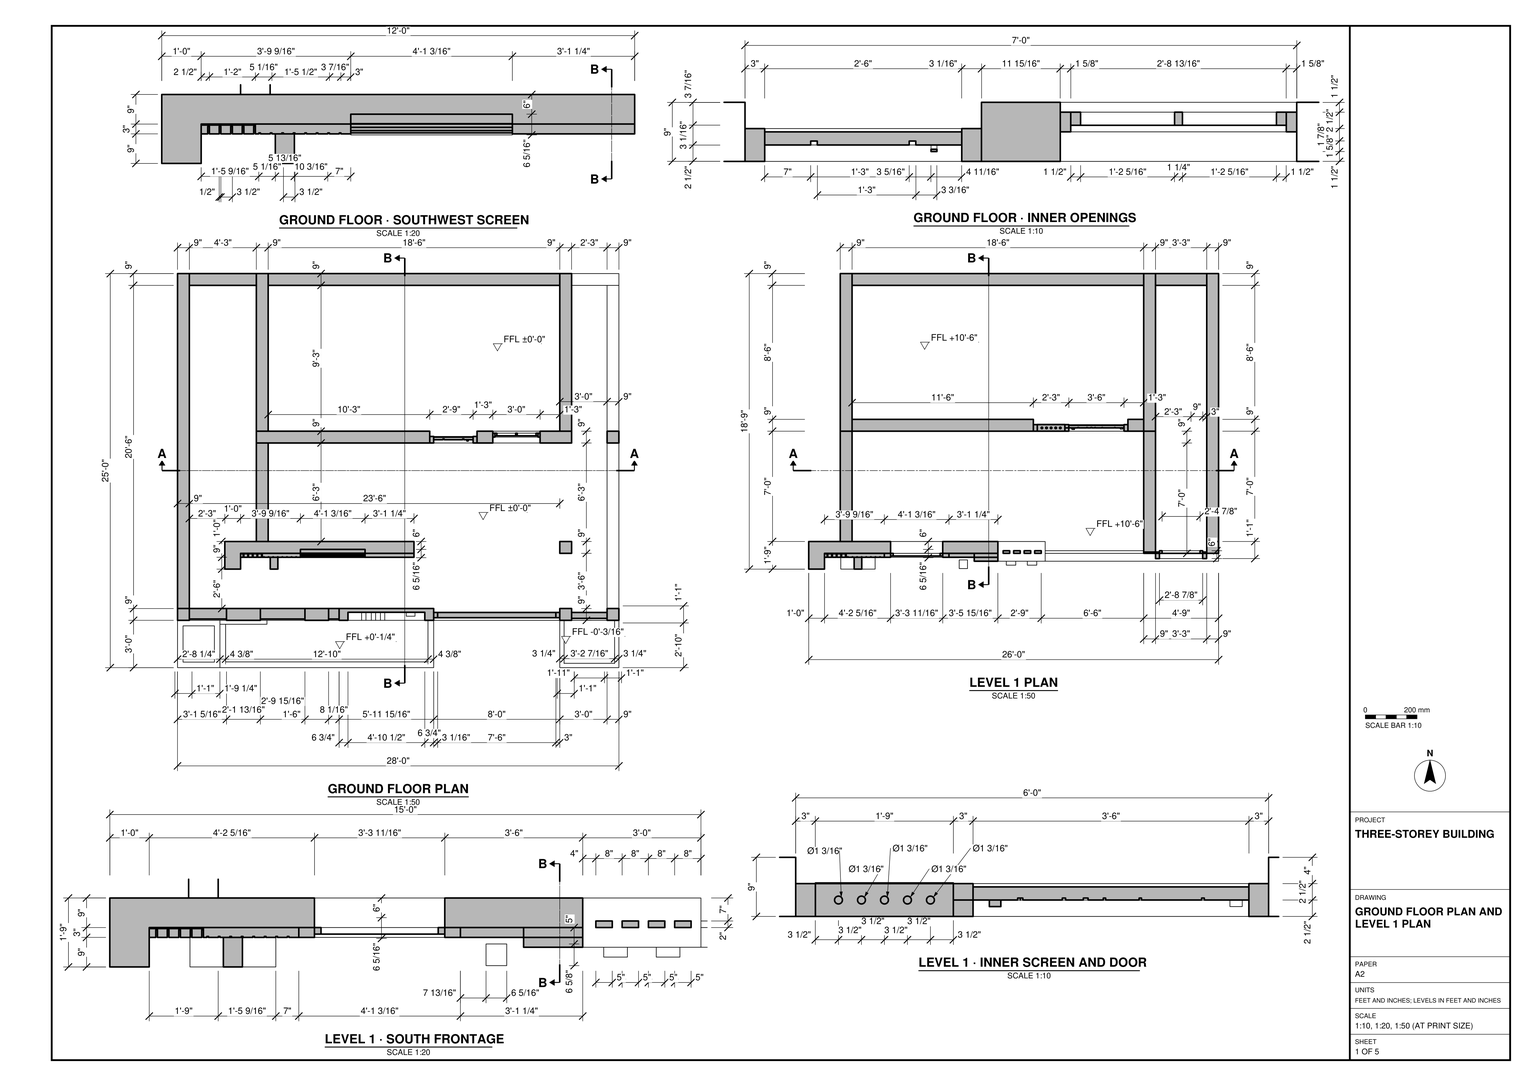
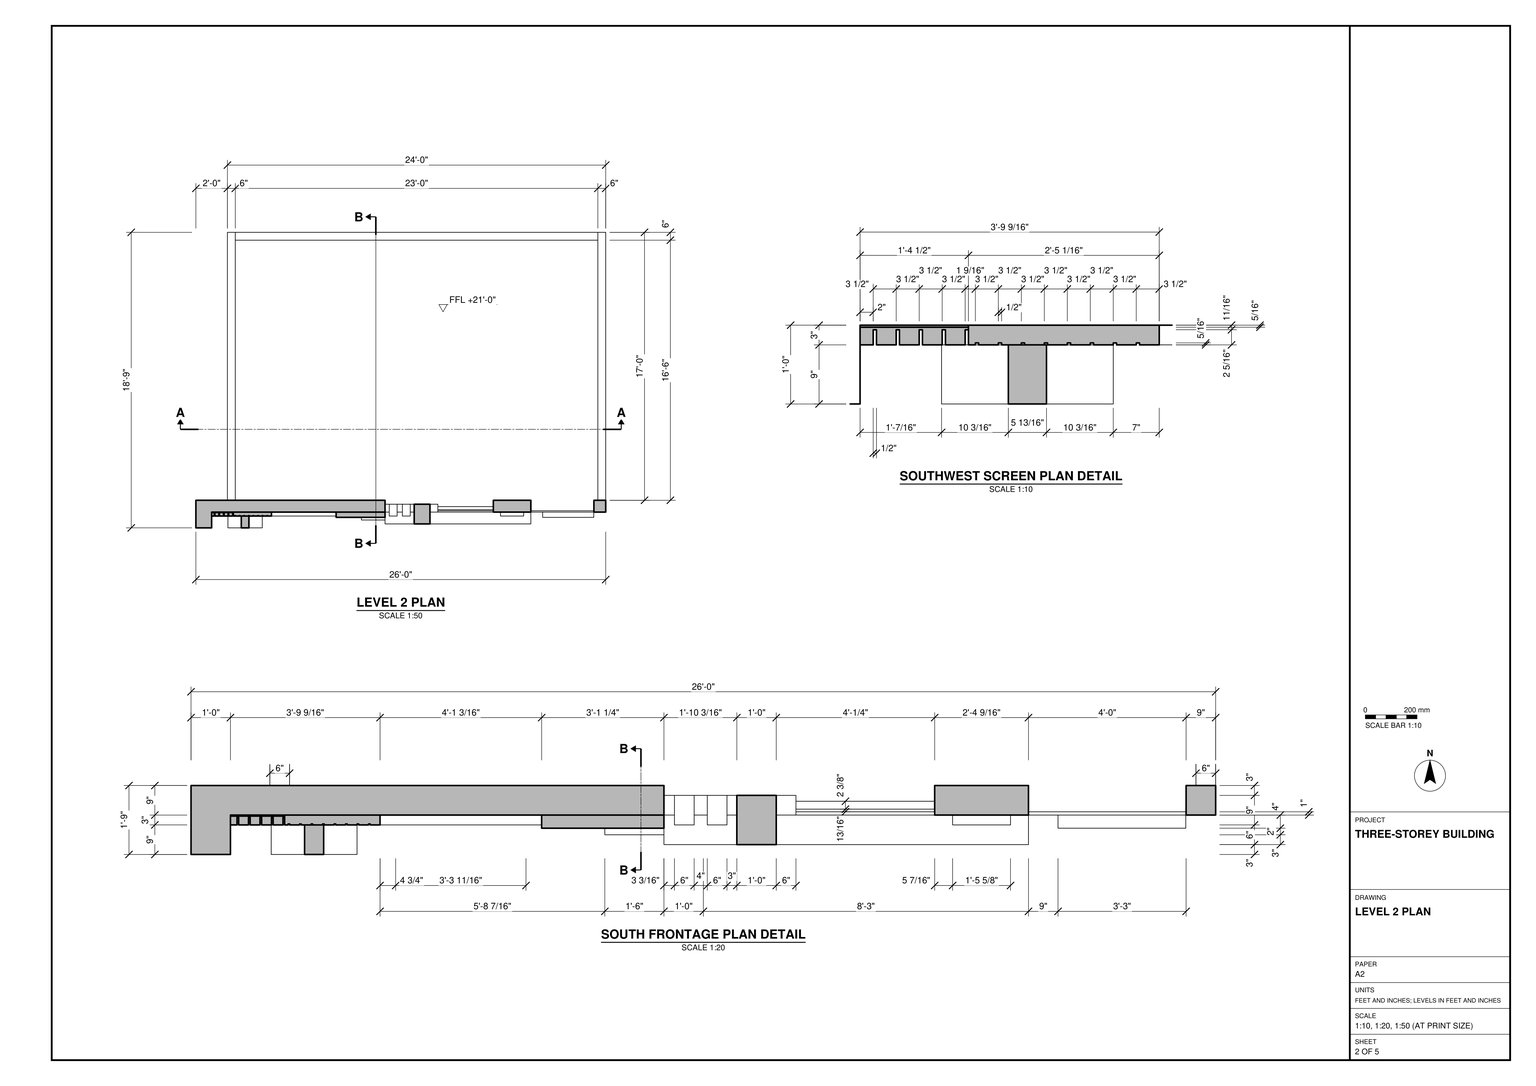
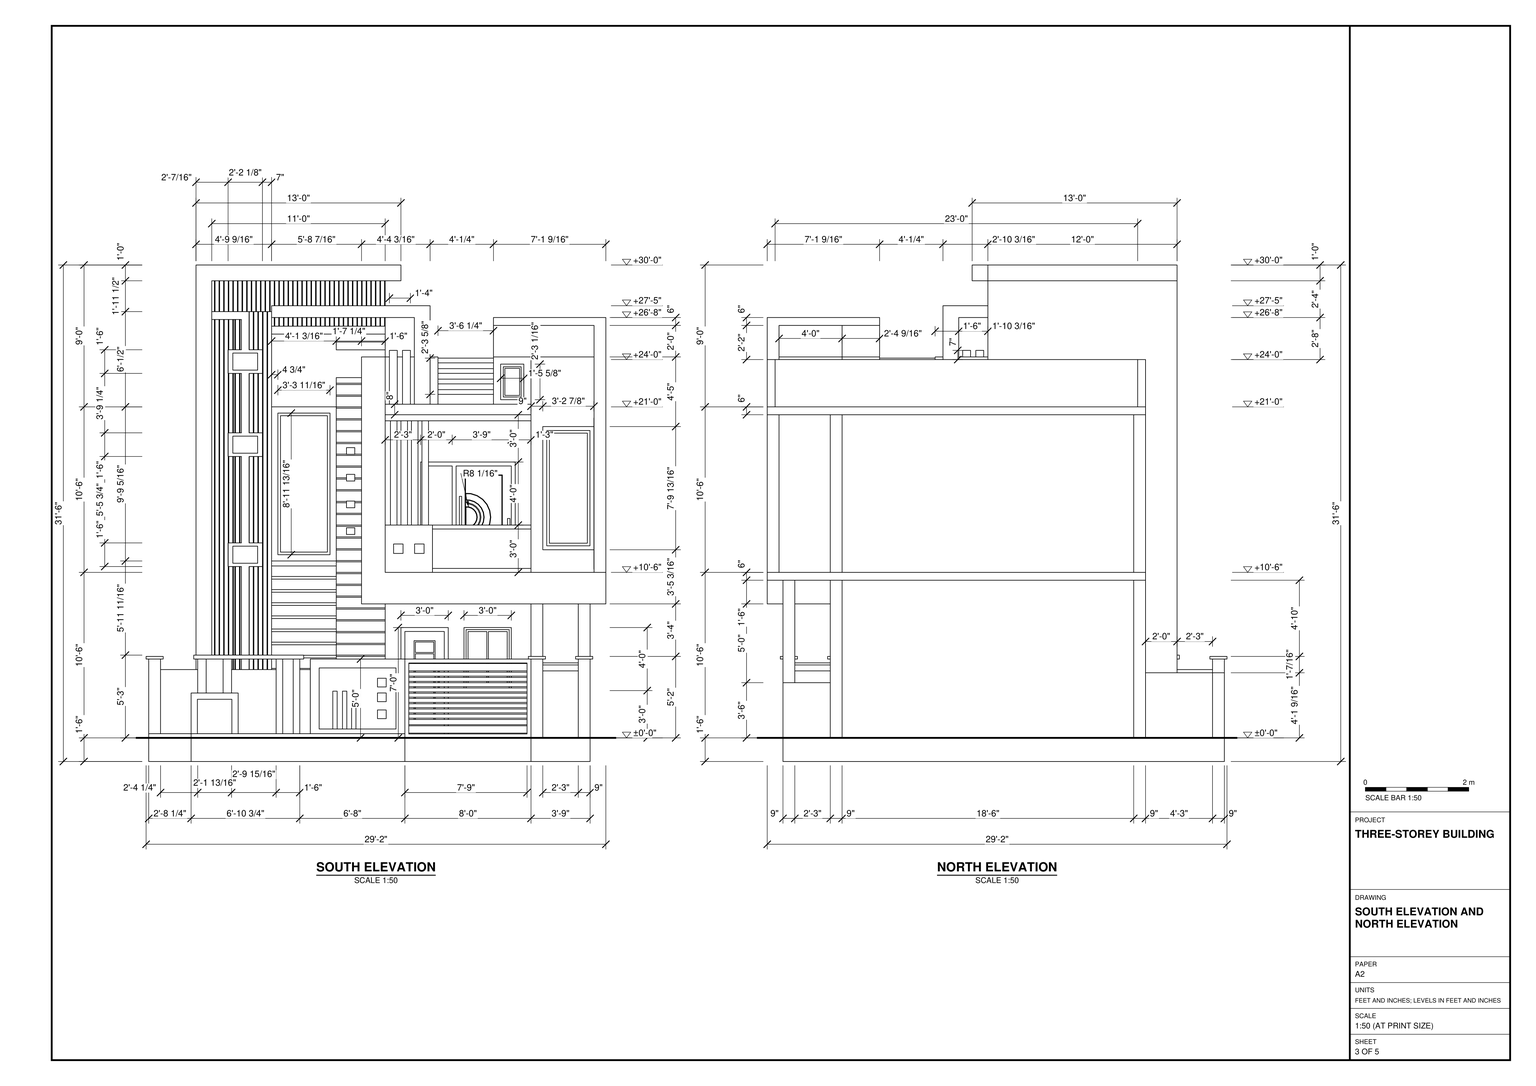
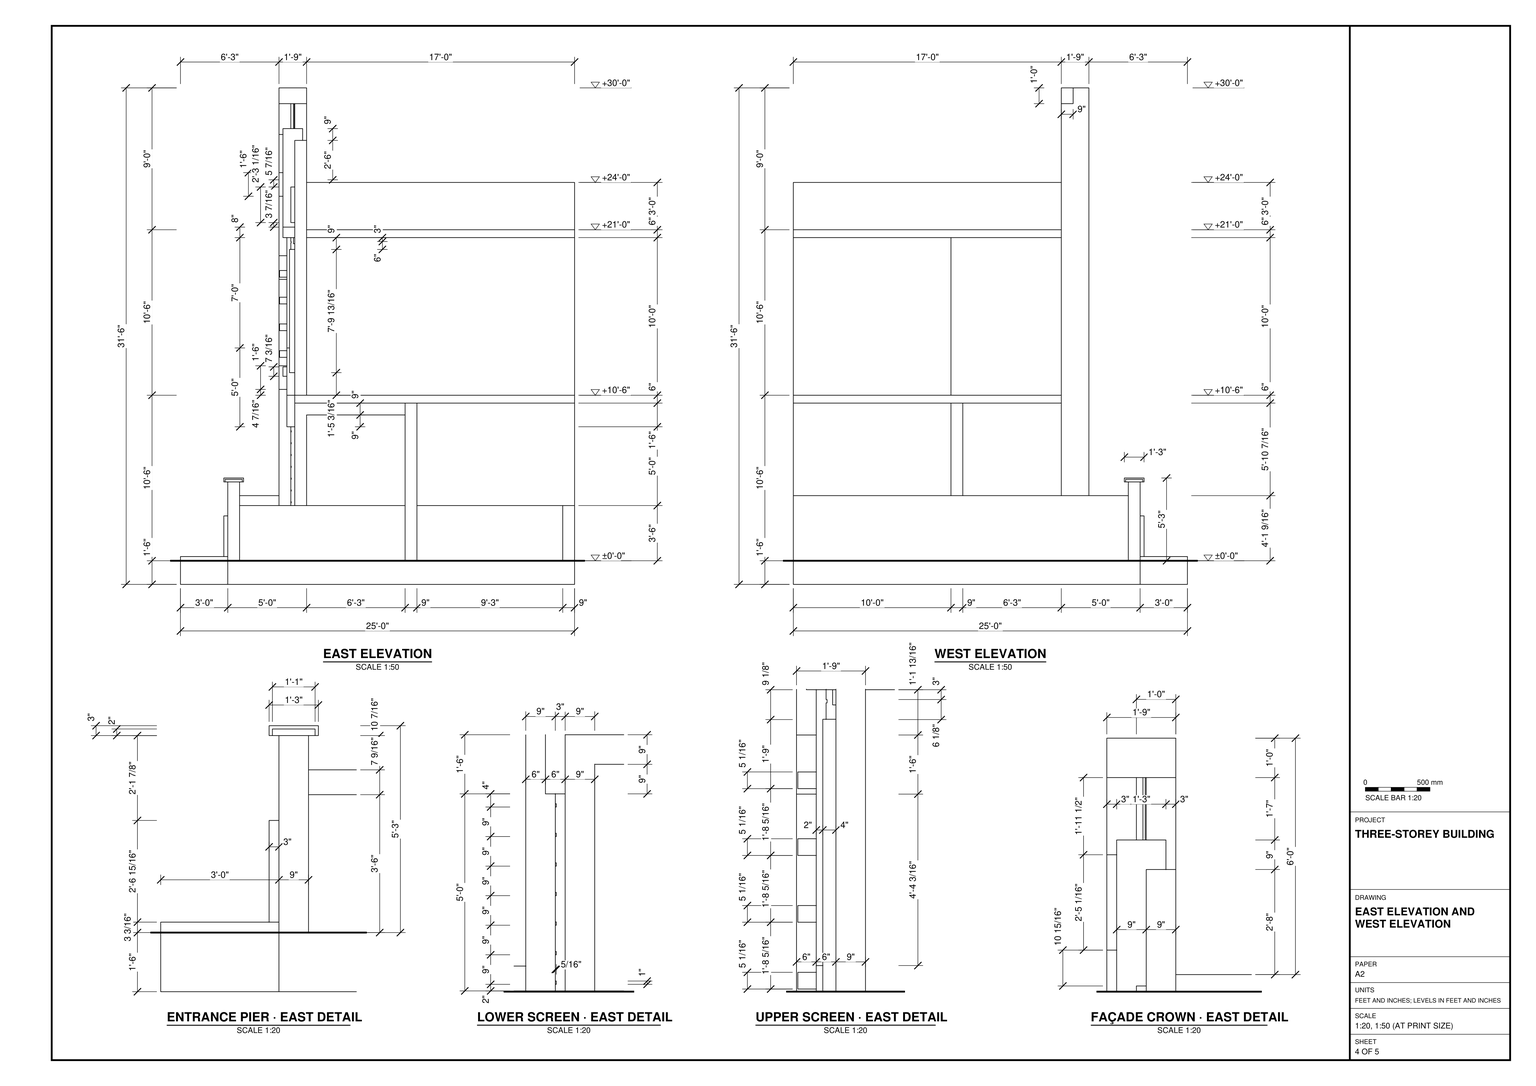
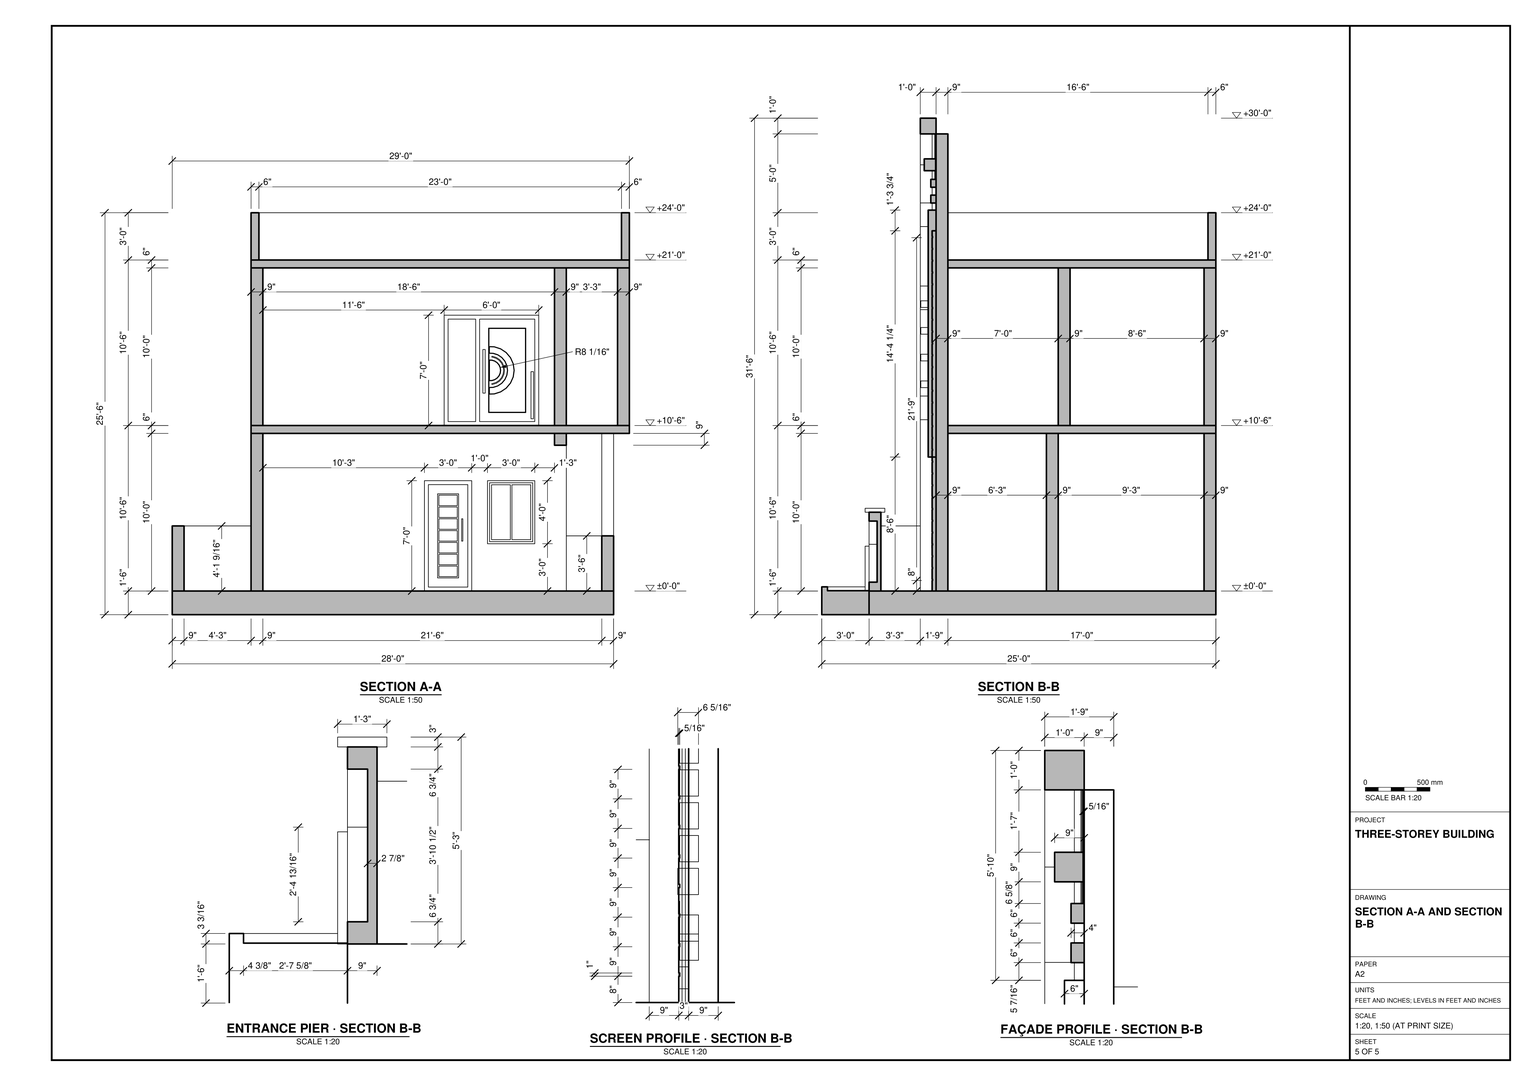
Build the three-storey building in SketchUp from task_files/diagram_01.pdf. Work in feet and inches. The overall model is 29'-2" east to west, 25'-0" north to south and 31'-6" high, including the base below the ground floor. Set the finished floor levels at ±0'-0", +10'-6" and +21'-0".

Use each floor plan to locate the slab edges, walls, piers and openings. Follow the wall thicknesses shown rather than extruding one perimeter through all three storeys. Model the inner openings in the ground-floor partition and the screen beside the level 1 door. Form the flat roof terrace with its low perimeter walls and the taller frames along its south edge.

Use the south elevation to align the ground-level gate, tall southwest screen, framed openings and recessed frontage above. Use the enlarged plan details to give the fins, frames and panels their different depths. Keep shell elements such as walls, slabs and roof, and each furniture or joinery piece shown, in separate groups or components. Use components for repeated parts. Decor and loose items may use any suitable library components. Save one SketchUp model as output_files/three_storey_building_with_a_screened_south_frontage.skp.

# SketchUp Ruby script. Lengths in inches.
U = 1.inch
M = Sketchup.active_model
def pt(a) = Geom::Point3d.new(a.map { |v| v * U })
def face(e, loops, mat)
  f = e.add_face(loops[0].map { |a| pt(a) })
  loops[1..].each { |l| e.add_face(l.map { |a| pt(a) }).erase! }
  f.material = f.back_material = mat if mat
  f
end
# faces: each face lists its corners as indices into pts; further lists are holes
def faces(e, pts, list, mat = nil) = list.each { |f| face(e, (f[0].is_a?(Array) ? f : [f]).map { |l| l.map { |i| pts[i] } }, mat) }
# xy, xz, yz: faces in a plane at the given z, y or x. An outline is a flat list of corners, or four numbers for a rectangle; further outlines are holes
def ring(l) = l.size == 4 ? [[l[0], l[1]], [l[2], l[1]], [l[2], l[3]], [l[0], l[3]]] : l.each_slice(2).to_a
def flat(e, list, mat, &to3) = list.each { |f| face(e, (f[0].is_a?(Array) ? f : [f]).map { |l| ring(l).map { |u, v| to3.(u, v) } }, mat) }
def xy(e, z, list, mat = nil) = flat(e, list, mat) { |x, y| [x, y, z] }
def xz(e, y, list, mat = nil) = flat(e, list, mat) { |x, z| [x, y, z] }
def yz(e, x, list, mat = nil) = flat(e, list, mat) { |y, z| [x, y, z] }
def lines(e, pts, list) = list.each { |a, b| e.add_line(pt(pts[a]), pt(pts[b])) }
# prism: a flat outline (further loops are holes) pulled along v
def prism(e, loops, v, mat = nil)
  f = face(e, loops, mat); d = Geom::Vector3d.new(v.map { |x| x * U })
  f.pushpull(f.normal.samedirection?(d) ? d.length : -d.length)
end
def box(e, o, s, mat = nil) = prism(e, [[o, [o[0] + s[0], o[1], o[2]], [o[0] + s[0], o[1] + s[1], o[2]], [o[0], o[1] + s[1], o[2]]]], [0, 0, s[2]], mat)
def at(x, y, z, deg = 0) = Geom::Transformation.translation(pt([x, y, z])) * Geom::Transformation.rotation(ORIGIN, Z_AXIS, deg.degrees)
def axes(o, x, y, z) = Geom::Transformation.new([*x, 0, *y, 0, *z, 0, *pt(o).to_a, 1])
def part(name) = M.definitions.add(name)
# library, detail: a bought-in or finely detailed component or shape, given as its bounding box
def library(name, o, s) = part(name).tap { |d| box(d.entities, o, s) }
def detail(e, o, s) = box(e.add_group.entities, o, s)
def put(e, d, t, mat = nil) = e.add_instance(d, t).tap { |i| i.material = mat if mat }
def group(e, t, mat = nil) = e.add_group.tap { |g| g.transformation = t; g.material = mat if mat }.entities
root = M.entities
M.materials.add("[0042_Sienna]").color = [160, 82, 45]
M.materials.add("[0137_Black]").color = [0, 0, 0]
M.materials.add("[Color E02]").color = [255, 255, 153]
M.materials.add("[Color M00]").color = [255, 255, 255]
M.materials.add("[Color M01]").color = [226, 226, 226]
M.materials.add("[Color M06]").color = [86, 86, 86]
M.materials.add("[Color M09]").color = [0, 0, 0]
M.materials.add("[Grass Dark Green]").color = [106, 157, 55]
M.materials.add("[Metal Aluminum Anodized]").color = [202, 209, 219]
M.materials.add("[Polished Concrete Old]").color = [229, 229, 229]
M.materials.add("[Translucent Glass Blue]").color = [65, 97, 155]
M.materials["[Translucent Glass Blue]"].alpha = 0.5
M.materials.add("[Wood Board Cork]").color = [158, 147, 84]
M.materials.add("[Wood Cherry Original]").color = [152, 86, 42]
M.materials.add("[Wood Veneer 01]").color = [120, 70, 37]
c1 = part("Group\#3")
box(c1.entities,[0,0,0],[9,120,120])
c2 = part("Group\#4")
box(c2.entities,[0,0,0],[9,120,120])
c3 = part("Group\#5")
box(c3.entities,[0,0,0],[222,9,120])
c4 = library("Group\#20",[-3,0,0],[45,2,78])
c5 = part("Group\#21")
prism(c5.entities,[[[0.59,0,0],[0.4375,0.02,0],[0.29,0.08,0],[0.17,0.18,0],[0.08,0.31,0],[0.02,0.45,0],[0,0.61,0],[0.02,0.76,0],[0.08,0.91,0],[0.18,1.03,0],[0.31,1.125,0],[0.45,1.18,0],[0.61,1.2,0],[0.76,1.18,0],[0.91,1.11,0],[1.03,1.02,0],[1.125,0.89,0],[1.18,0.75,0],[1.2,0.59,0],[1.18,0.4375,0],[1.11,0.29,0],[1.02,0.17,0],[0.89,0.08,0],[0.75,0.02,0]]],[0,0,78])
c6 = part("Group\#23")
prism(c6.entities,[[[21,0.5,0.79],[21,0.4,0.8],[21,0.29,0.79],[21,0.2,0.74],[21,0.11,0.68],[21,0.05,0.6],[21,0.01,0.5],[21,0,0.4],[21,0.01,0.29],[21,0.06,0.2],[21,0.12,0.11],[21,0.2,0.05],[21,0.3,0.01],[21,0.4,0],[21,0.51,0.01],[21,0.6,0.06],[21,0.69,0.12],[21,0.75,0.2],[21,0.79,0.3],[21,0.8,0.4],[21,0.79,0.51],[21,0.74,0.6],[21,0.68,0.69],[21,0.6,0.75]]],[-21,0,0])
c7 = part("Group\#46")
box(c7.entities,[0,0,0],[52.8,2.4,3.6])
c8 = part("Group\#50")
box(c8.entities,[0,0,0],[5,2,84])
c9 = library("Group\#58",[-12,-2,-320],[132,2.6875,348])
c10 = part("Group\#65")
box(c10.entities,[0,0,0],[5.125,2,4.5])
c11 = part("Group\#82")
box(c11.entities,[0,0,0],[6.625,3,6.625])
c12 = part("Group\#84")
box(c12.entities,[0,0,0],[90,4,5.6])
c13 = part("Group\#86")
box(c13.entities,[0,0,0],[90,4,3])
xy(root,308.37,[[264.44,87,293,96]])
xy(root,332.37,[[264.44,87,293,96]])
xz(root,85,[[102.3125,159.81,138,263.62]],"[Translucent Glass Blue]")
xz(root,86,[[273.125,279.06,284.32,299.6875]],"[Translucent Glass Blue]")
xz(root,87,[[264.44,308.37,293,332.37]],"[Color M00]")
xz(root,96,[[264.44,308.37,293,332.37]])
xz(root,180,[[212,147.37,233,225.37]],"[Translucent Glass Blue]")
yz(root,264.44,[[87,308.37,96,332.37]])
yz(root,293,[[87,308.37,96,332.37]])
p = [[95.55,86,347.37],[182,86,347.37],[182,87,347.37],[95.55,86,338.37],[182,86,338.37]]
lines(root,p,[[0,1],[1,2],[3,4]])
g1 = group(root,at(62,60,12.37))
box(g1,[-60,-24,-12],[336,264,18])
g2 = group(root,at(62,171,18.37),"[Color M00]")
prism(g2,[[[240,9,0],[168,9,0],[168,9,84],[132,9,84],[132,9,0],[0,9,0],[0,9,120],[240,9,120]],[[216,9,84],[180,9,84],[180,9,36],[216,9,36]]],[0,-9,0])
put(root,c1,at(293,180,18.37),"[Color M00]")
put(root,c2,at(62,180,18.37),"[Color M00]")
put(root,c3,at(71,291,18.37),"[Color M00]")
g3 = group(root,at(194,171,18.37),"[Wood Veneer 01]")
prism(g3,[[[0,5,0],[0,5,84],[36,5,84],[36,5,0]],[[3,5,81],[3,5,3],[33,5,3],[33,5,81]]],[0,-5,0])
g4 = group(root,at(197,173.5,21.37),"[Wood Veneer 01]")
xy(g4,0,[[0,0,30,2]])
xy(g4,7,[[7,0,23,0.6]])
xy(g4,8,[[8,0,22,0.6]])
xy(g4,16,[[8,0,22,0.6]])
xy(g4,17,[[8,0,22,0.6]])
xy(g4,25,[[8,0,22,0.6]])
xy(g4,26,[[8,0,22,0.6]])
xy(g4,34,[[8,0,22,0.6]])
xy(g4,35,[[8,0,22,0.6]])
xy(g4,43,[[8,0,22,0.6]])
xy(g4,44,[[8,0,22,0.6]])
xy(g4,52,[[8,0,22,0.6]])
xy(g4,53,[[8,0,22,0.6]])
xy(g4,61,[[8,0,22,0.6]])
xy(g4,62,[[8,0,22,0.6]])
xy(g4,70,[[8,0,22,0.6]])
xy(g4,71,[[7,0,23,0.6]])
xy(g4,78,[[0,0,30,2]])
xz(g4,0,[[[0,0,30,78],[7,7,23,71]],[8,8,22,16],[8,17,22,25],[8,26,22,34],[8,35,22,43],
  [8,44,22,52],[8,53,22,61],[8,62,22,70]])
xz(g4,0.6,[[[7,7,23,71],[8,8,22,16],[8,62,22,70],[8,17,22,25],[8,44,22,52],[8,53,22,61],[8,26,22,34],[8,35,22,43]]])
xz(g4,2,[[0,0,30,78]])
yz(g4,0,[[0,0,2,78]])
yz(g4,7,[[0,7,0.6,71]])
yz(g4,8,[[0,8,0.6,16],[0,17,0.6,25],[0,26,0.6,34],[0,35,0.6,43],[0,44,0.6,52],
  [0,53,0.6,61],[0,62,0.6,70]])
yz(g4,22,[[0,8,0.6,16],[0,17,0.6,25],[0,26,0.6,34],[0,35,0.6,43],[0,44,0.6,52],
  [0,53,0.6,61],[0,62,0.6,70]])
yz(g4,23,[[0,7,0.6,71]])
yz(g4,30,[[0,0,2,78]])
g5 = group(root,at(222.32,172.5,56.37),"[Metal Aluminum Anodized]")
prism(g5,[[[0,1,17],[0,1,16.65],[0,0.35,16.65],[0,0.35,0.35],[0,1,0.35],[0,1,0],[0,0,0],[0,0,17]]],[0.9,0,0])
g6 = group(root,at(242,175.5,54.37),"[Color M09]")
g7 = group(g6,at(1.59,1,1.59))
prism(g7,[[[32.82,2,0],[0,2,0],[0,2,44.82],[32.82,2,44.82]],[[1.5,2,1.5],[15.81,2,1.5],[15.81,2,43.32],[1.5,2,43.32]],[[17.01,2,43.32],[17.01,2,1.5],[31.32,2,1.5],[31.32,2,43.32]]],[0,-2,0])
g8 = group(g6,at(0,0,0))
prism(g8,[[[0,3,48],[36,3,48],[36,3,0],[0,3,0]],[[1.59,3,46.41],[1.59,3,1.59],[34.41,3,1.59],[34.41,3,46.41]]],[0,-3,0])
g9 = group(root,at(260.6,176.5,57.46),"[Translucent Glass Blue]")
xz(g9,0,[[0,0,14.31,41.82]])
g10 = group(root,at(245.09,176.5,57.46),"[Translucent Glass Blue]")
xz(g10,0,[[0,0,14.31,41.82]])
g11 = group(root,at(293,87,18.37),"[Color M00]")
prism(g11,[[[0,9,0],[0,0,0],[0,0,120],[0,84,120],[0,84,111],[0,9,111]]],[9,0,0])
g12 = group(root,at(329,171,18.37),"[Color M00]")
box(g12,[0,0,0],[9,9,120])
g13 = group(root,at(62,87,18.37),"[Color M00]")
xy(g13,0,[[-24,-12,-24,9,120,9,120,0,-12,0,-12,-12]])
xy(g13,139.4375,[[38.3125,0,78,9]])
xy(g13,247.25,[[38.3125,0,78,9]])
xy(g13,348,[[-12,-12,-12,0,120,0,120,9,132,9,132,-12],[-24,0,120,9]])
xy(g13,360,[[-24,-12,132,-12,132,9,120,9,120,0,-24,0]])
xz(g13,-12,[[-24,0,-12,0,-12,348,132,348,132,360,-24,360]])
xz(g13,0,[[[-12,0,120,348],[38.3125,139.4375,78,247.25]],[-24,348,120,360]])
xz(g13,9,[[[-24,0,120,348],[38.3125,139.4375,78,247.25]],[120,348,132,360]])
yz(g13,-24,[[-12,0,-12,360,0,360,0,348,9,348,9,0]])
yz(g13,-12,[[-12,0,0,348]])
yz(g13,38.3125,[[0,139.4375,9,247.25]])
yz(g13,78,[[0,139.4375,9,247.25]])
yz(g13,120,[[0,0,9,348],[0,348,9,360]])
yz(g13,132,[[-12,348,9,360]])
put(root,c3,at(71,291,144.37),"[Color M00]")
put(root,c1,at(293,180,144.37),"[Color M00]")
put(root,c2,at(62,180,144.37),"[Color M00]")
g14 = group(root,at(62,87,138.37),"[Color M00]")
prism(g14,[[[288,213,0],[288,0,0],[120,0,0],[120,9,0],[0,9,0],[0,213,0]]],[0,0,6])
g15 = group(root,at(71,180,144.37),"[Color M00]")
prism(g15,[[[138,9,0],[0,9,0],[0,9,120],[222,9,120],[222,9,0],[210,9,0],[210,9,84],[138,9,84]]],[0,-9,0])
g16 = group(root,at(209,180,144.37),"[Wood Veneer 01]")
prism(g16,[[[0,0,0],[72,0,0],[72,0,84],[0,0,84]],[[69,0,81],[69,0,3],[27,0,3],[27,0,81]],[[24,0,3],[3,0,3],[3,0,81],[24,0,81]]],[0,5,0])
put(root,c4,at(236,182.5,147.37),"[Wood Veneer 01]")
g17 = group(root,at(214.91,181.9,147.37))
put(g17,c5,at(14,0,0))
put(g17,c5,at(10.5,0,0))
put(g17,c5,at(7,0,0))
put(g17,c5,at(0,0,0))
put(g17,c5,at(3.5,0,0))
put(root,c6,at(212,182.1,150.92))
put(root,c6,at(212,182.1,159.92))
put(root,c6,at(212,182.1,168.92))
put(root,c6,at(212,182.1,177.92))
put(root,c6,at(212,182.1,186.92))
put(root,c6,at(212,182.1,195.92))
put(root,c6,at(212,182.1,204.92))
put(root,c6,at(212,182.1,213.92))
put(root,c6,at(212,182.1,222.92))
put(root,c6,at(212,182.1,231.92))
g18 = group(root,at(212,185,147.37))
box(g18,[0,0,0],[21,0.1,78])
g19 = group(root,at(62,180,264.37),"[Color M00]")
prism(g19,[[[231,-92,0],[231,-93,0],[120,-93,0],[120,-84,0],[0,-84,0],[0,120,0],[288,120,0],[288,-84,0],[279,-84,0],[279,-92,0]]],[0,0,6])
g20 = group(root,at(62,96,18.37),"[Color M00]")
box(g20,[0,0,0],[9,75,120])
g21 = group(root,at(62,96,144.37),"[Color M00]")
box(g21,[0,0,0],[9,84,120])
g22 = group(root,at(293,87,144.37),"[Color M00]")
box(g22,[0,1,0],[9,92,120])
g23 = group(root,at(182,87,144.37),"[Color M00]")
box(g23,[0,-6,0],[36,15,36])
g24 = group(root,at(218,87,144.37))
box(g24,[0,0,0],[75,2,3])
g25 = group(root,at(218,87,177.37))
box(g25,[0,0,0],[75,2,3])
g26 = group(root,at(218,87.1875,147.37),"[Translucent Glass Blue]")
xz(g26,0,[[0,0,75,30]])
g27 = group(root,at(341,87,144.37),"[Color M00]")
prism(g27,[[[-76.56,9,194],[9,9,194],[9,9,0],[0,9,0],[0,9,188],[-76.56,9,188]]],[0,-9,0])
g28 = group(root,at(293,87,144.37),"[Polished Concrete Old]")
xy(g28,0,[[0,0,48,1]])
xy(g28,2.46,[[47.9,0,48,1]])
xy(g28,20.21,[[12,0,44.9,1]])
xy(g28,108,[[12,0,44.9,1],[44.9,0,47.9,1]])
xy(g28,117.54,[[47.9,0,48,1]])
xy(g28,164,[[0,0,48,1]])
xz(g28,0,[[0,0,48,0,48,117.54,47.9,117.54,47.9,108,44.9,108,44.9,20.21,12,20.21,12,108,47.9,108,47.9,117.54,48,117.54,48,164,0,164]])
xz(g28,1,[[0,0,0,164,48,164,48,117.54,47.9,117.54,47.9,108,12,108,12,20.21,47.9,20.21,47.9,2.46,48,2.46,48,0],[47.9,2.46,47.9,20.21,44.9,20.21,44.9,108,47.9,108,47.9,117.54,48,117.54,48,2.46]])
yz(g28,0,[[0,0,1,164]])
yz(g28,12,[[0,20.21,1,108]])
yz(g28,44.9,[[0,20.21,1,108]])
yz(g28,47.9,[[0,2.46,1,20.21],[0,108,1,117.54]])
yz(g28,48,[[0,0,1,2.46],[0,2.46,1,117.54],[0,117.54,1,164]])
g29 = group(root,at(302,83,161.58),"[Color M00]")
prism(g29,[[[0,4,0],[0,4,93.79],[38.9,4,93.79],[38.9,4,0]],[[35.9,4,90.79],[3,4,90.79],[3,4,3],[35.9,4,3]]],[0,-4,0])
g30 = group(root,at(305,85,164.58),"[0137_Black]")
prism(g30,[[[0,4,0],[0,4,87.79],[32.9,4,87.79],[32.9,4,0]],[[30.9,4,2],[30.9,4,85.79],[2,4,85.79],[2,4,2]]],[0,-2,0])
g31 = group(root,at(307,87,166.58),"[Translucent Glass Blue]")
xz(g31,0,[[0,0,28.9,83.79]])
g32 = group(root,at(182,81,264.37),"[Color M00]")
box(g32,[0,-3,0],[111,9,8])
g33 = group(root,at(195.2,84,272.37),"[Color M06]")
prism(g33,[[[6,3,0],[6,3,34],[6,3,36],[6,9,36],[6,9,41],[6,0,41],[6,0,0]]],[-6,0,0])
g34 = group(root,at(185.2,84,272.37),"[Color M06]")
prism(g34,[[[0,3,34],[0,3,0],[0,0,0],[0,0,41],[0,9,41],[0,9,36],[0,3,36]]],[6,0,0])
g35 = group(root,at(216.2,87,270.37))
box(g35,[0,0,0],[6,6,38],"[Color M06]")
g36 = group(root,at(275,87,270.37),"[Color M00]")
prism(g36,[[[18,9,0],[-10.56,9,0],[-10.56,9,38],[18,9,38]],[[10.5,9,7.5],[10.5,9,30.5],[-3.06,9,30.5],[-3.06,9,7.5]]],[0,-9,0])
g37 = group(root,at(222.2,87,270.37),"[Color M00]")
box(g37,[0,0,0],[42.24,1,9.5])
g38 = group(root,at(182,87,270.37))
box(g38,[0,0,0],[22.2,6,38],"[Color E02]")
g39 = group(root,at(222.2,88.8,279.87),"[Color M06]")
put(g39,c7,axes([0,0,16],[0.8,0,0],[0,1,0],[0,0,1]))
put(g39,c7,axes([0,0,8],[0.8,0,0],[0,1,0],[0,0,1]))
put(g39,c7,axes([0,0,0],[0.8,0,0],[0,1,0],[0,0,1]))
put(g39,c7,axes([0,0,24],[0.8,0,0],[0,1,0],[0,0,1]))
g40 = group(root,at(269.9,84,275.84))
prism(g40,[[[17.64,3,27.08],[17.64,3,0],[0,3,0],[0,3,27.08]],[[2.04,3,25.04],[2.04,3,2.04],[15.6,3,2.04],[15.6,3,25.04]]],[0,-3,0])
g41 = group(root,at(271.94,86,277.87),"[0137_Black]")
prism(g41,[[[13.5625,1,23],[13.5625,1,0],[0,1,0],[0,1,23]],[[1.18,1,21.82],[1.18,1,1.18],[12.375,1,1.18],[12.375,1,21.82]]],[0,-1,0])
put(root,c8,at(186,87,180.37),"[Wood Veneer 01]")
put(root,c8,at(194,87,180.37),"[Wood Veneer 01]")
put(root,c8,at(202,87,180.37),"[Wood Veneer 01]")
put(root,c8,at(210,87,180.37),"[Wood Veneer 01]")
g42 = group(root,at(188.4,78,158.77),"[Color E02]")
box(g42,[0,0,0],[7.2,3,7.2])
g43 = group(root,at(204.4,78,158.77),"[Color E02]")
box(g43,[0,0,0],[7.2,3,7.2])
g44 = group(root,at(95.55,84,153.05))
prism(g44,[[[49.21,3,117.33],[49.21,3,0],[0,3,0],[0,3,117.33]],[[4.76,3,4.76],[44.45,3,4.76],[44.45,3,112.57],[4.76,3,112.57]]],[0,-3,0])
g45 = group(root,at(100.3125,85,157.81),"[Color M09]")
prism(g45,[[[0,2,0],[0,2,107.8125],[39.6875,2,107.8125],[39.6875,2,0]],[[2,2,105.8125],[2,2,2],[37.6875,2,2],[37.6875,2,105.8125]]],[0,-2,0])
g46 = group(root,at(164,81,120.37),"[Color M06]")
xy(g46,0,[[0,0,186,6]])
xy(g46,24,[[18,0,186,6]])
xy(g46,188,[[0,0,18,6]])
xz(g46,0,[[0,0,186,0,186,24,18,24,18,188,0,188]])
xz(g46,6,[[0,0,0,188,18,188,18,24,186,24,186,0]])
yz(g46,0,[[0,0,0,188,6,188,6,172.25,3,172.25,3,0],[3,0,6,172.25]])
yz(g46,18,[[0,24,6,188]])
yz(g46,186,[[0,0,6,24]])
p = [[18,3,0],[0,3,0]]
lines(g46,p,[[0,1]])
g47 = group(root,at(182,86,259.75),"[0042_Sienna]")
box(g47,[0,0,0],[111,1,4.62])
g48 = group(root,at(144.76,84,18.37),"[Color M06]")
prism(g48,[[[37.24,3,0],[37.24,3,274.25],[37.24,0,274.25],[37.24,0,270],[37.24,0.3,270],[37.24,0.3,269],[37.24,0,269],[37.24,0,261],[37.24,0.3,261],[37.24,0.3,260],[37.24,0,260],[37.24,0,252],[37.24,0.3,252],[37.24,0.3,251],[37.24,0,251],[37.24,0,243],[37.24,0.3,243],[37.24,0.3,242],[37.24,0,242],[37.24,0,234],[37.24,0.3,234],[37.24,0.3,233],[37.24,0,233],[37.24,0,225],[37.24,0.3,225],[37.24,0.3,224],[37.24,0,224],[37.24,0,216],[37.24,0.3,216],[37.24,0.3,215],[37.24,0,215],[37.24,0,207],[37.24,0.3,207],[37.24,0.3,206],[37.24,0,206],[37.24,0,198],[37.24,0.3,198],[37.24,0.3,197],[37.24,0,197],[37.24,0,189],[37.24,0.3,189],[37.24,0.3,188],[37.24,0,188],[37.24,0,180],[37.24,0.3,180],[37.24,0.3,179],[37.24,0,179],[37.24,0,171],[37.24,0.3,171],[37.24,0.3,170],[37.24,0,170],[37.24,0,162],[37.24,0.3,162],[37.24,0.3,161],[37.24,0,161],[37.24,0,153],[37.24,0.3,153],[37.24,0.3,152],[37.24,0,152],[37.24,0,144],[37.24,0.3,144],[37.24,0.3,143],[37.24,0,143],[37.24,0,135],[37.24,0.3,135],[37.24,0.3,134],[37.24,0,134],[37.24,0,126],[37.24,0.3,126],[37.24,0.3,125],[37.24,0,125],[37.24,0,117],[37.24,0.3,117],[37.24,0.3,116],[37.24,0,116],[37.24,0,108],[37.24,0.3,108],[37.24,0.3,107],[37.24,0,107],[37.24,0,99],[37.24,0.3,99],[37.24,0.3,98],[37.24,0,98],[37.24,0,90],[37.24,0.3,90],[37.24,0.3,89],[37.24,0,89],[37.24,0,81],[37.24,0.3,81],[37.24,0.3,80],[37.24,0,80],[37.24,0,72],[37.24,0.3,72],[37.24,0.3,71],[37.24,0,71],[37.24,0,63],[37.24,0.3,63],[37.24,0.3,62],[37.24,0,62],[37.24,0,54],[37.24,0.3,54],[37.24,0.3,53],[37.24,0,53],[37.24,0,45],[37.24,0.3,45],[37.24,0.3,44],[37.24,0,44],[37.24,0,36],[37.24,0.3,36],[37.24,0.3,35],[37.24,0,35],[37.24,0,27],[37.24,0.3,27],[37.24,0.3,26],[37.24,0,26],[37.24,0,18],[37.24,0.3,18],[37.24,0.3,17],[37.24,0,17],[37.24,0,9],[37.24,0.3,9],[37.24,0.3,8],[37.24,0,8],[37.24,0,0]]],[-37.24,0,0])
g49 = group(root,at(204.2,87,270.37),"[Color M06]")
xy(g49,2,[[0,-9,12,6]])
xy(g49,68,[[-108.65,-9,-108.65,0,-22.2,0,-22.2,6,0,6,0,-9]])
xy(g49,77,[[-108.65,-9,12,-9,12,6,-22.2,6,-22.2,0,-108.65,0]])
xz(g49,-9,[[0,2,12,2,12,77,-108.65,77,-108.65,68,0,68]])
xz(g49,0,[[-108.65,68,-22.2,77]])
xz(g49,6,[[0,2,0,68,-22.2,68,-22.2,77,12,77,12,2]])
yz(g49,-108.65,[[-9,68,0,77]])
yz(g49,-22.2,[[0,68,6,77]])
yz(g49,0,[[-9,2,6,68]])
yz(g49,12,[[-9,2,6,77]])
put(root,c9,at(62,86,338.37),"[Wood Cherry Original]")
g50 = group(root,at(66.5,84,18.37),"[Color M06]")
xy(g50,0,[[0,0,0,3,29.05,3,29.05,0,26.05,0,26.05,0.3,25.55,0.3,25.55,0,22.55,0,22.55,0.3,22.05,0.3,22.05,0,19.05,0,19.05,0.3,18.55,0.3,18.55,0,15.55,0,15.55,0.3,15.05,0.3,15.05,0,12.05,0,12.05,0.3,11.55,0.3,11.55,0,8.55,0,8.55,0.3,8.05,0.3,8.05,0,5.05,0,5.05,0.3,4.55,0.3,4.55,0,1.55,0,1.55,0.3,1.05,0.3,1.05,0]])
xy(g50,320,[[0,2,29.05,3]])
xy(g50,324.5,[[0,0,1.05,0,1.05,0.3,1.55,0.3,1.55,0,4.55,0,4.55,0.3,5.05,0.3,5.05,0,8.05,0,8.05,0.3,8.55,0.3,8.55,0,11.55,0,11.55,0.3,12.05,0.3,12.05,0,15.05,0,15.05,0.3,15.55,0.3,15.55,0,18.55,0,18.55,0.3,19.05,0.3,19.05,0,22.05,0,22.05,0.3,22.55,0.3,22.55,0,25.55,0,25.55,0.3,26.05,0.3,26.05,0,29.05,0,29.05,2,0,2]])
xz(g50,0,[[0,0,1.05,324.5],[1.55,0,4.55,324.5],[5.05,0,8.05,324.5],[8.55,0,11.55,324.5],[12.05,0,15.05,324.5],
  [15.55,0,18.55,324.5],[19.05,0,22.05,324.5],[22.55,0,25.55,324.5],[26.05,0,29.05,324.5]])
xz(g50,0.3,[[1.05,0,1.55,324.5],[4.55,0,5.05,324.5],[8.05,0,8.55,324.5],[11.55,0,12.05,324.5],[15.05,0,15.55,324.5],
  [18.55,0,19.05,324.5],[22.05,0,22.55,324.5],[25.55,0,26.05,324.5]])
xz(g50,2,[[0,320,29.05,324.5]])
xz(g50,3,[[0,0,29.05,320]])
yz(g50,0,[[0,0,0,324.5,2,324.5,2,320,3,320,3,0]])
yz(g50,1.05,[[0,0,0.3,324.5]])
yz(g50,1.55,[[0,0,0.3,324.5]])
yz(g50,4.55,[[0,0,0.3,324.5]])
yz(g50,5.05,[[0,0,0.3,324.5]])
yz(g50,8.05,[[0,0,0.3,324.5]])
yz(g50,8.55,[[0,0,0.3,324.5]])
yz(g50,11.55,[[0,0,0.3,324.5]])
yz(g50,12.05,[[0,0,0.3,324.5]])
yz(g50,15.05,[[0,0,0.3,324.5]])
yz(g50,15.55,[[0,0,0.3,324.5]])
yz(g50,18.55,[[0,0,0.3,324.5]])
yz(g50,19.05,[[0,0,0.3,324.5]])
yz(g50,22.05,[[0,0,0.3,324.5]])
yz(g50,22.55,[[0,0,0.3,324.5]])
yz(g50,25.55,[[0,0,0.3,324.5]])
yz(g50,26.05,[[0,0,0.3,324.5]])
yz(g50,29.05,[[0,0,3,0,3,320,2,320,2,324.5,0,324.5]])
g51 = group(root,at(95.55,83,325.77),"[Color M06]")
box(g51,[0,0,0],[86.45,4,6])
g52 = group(root,at(140.61,83,313.77),"[Color M06]")
box(g52,[4.16,0,0],[37.23,4,6])
g53 = group(root,at(95.55,87,18.37),"[Color E02]")
box(g53,[0,0,0],[49.21,0.1,134.68])
g54 = group(root,at(95.55,83.6875,22.56),"[Color M06]")
box(g54,[0,0.61,48.68],[49.21,5.7,8])
box(g54,[0,0.61,58.68],[49.21,5.7,8])
box(g54,[0,0.61,38.68],[49.21,5.7,8])
box(g54,[0,0.3125,88.68],[49.21,6,8])
box(g54,[0,0.61,68.68],[49.21,5.7,8])
box(g54,[0,0.61,118.68],[49.21,5.7,8])
box(g54,[0,0.61,98.68],[49.21,5.7,8])
box(g54,[0,0.61,108.68],[49.21,5.7,8])
box(g54,[0,0.3125,78.68],[49.21,6,8])
box(g54,[0,0.61,8.68],[49.21,5.7,8])
box(g54,[0,0.3125,0],[49.21,3,6.68])
box(g54,[0,0,28.68],[49.21,6.3125,8])
xz(g54,0.61,[[0,18.68,49.21,26.68]])
g55 = group(root,at(62.41,75,18.37))
prism(g55,[[[10.17,0,295.46],[0,0,295.46],[0,0,277.46],[10.17,0,277.46],[10.17,0,232.21],[0,0,232.21],[0,0,214.21],[10.17,0,214.21],[10.17,0,148.4375],[0,0,148.4375],[0,0,130.4375],[10.17,0,130.4375],[10.17,0,0],[15.98,0,0],[15.98,0,130.4375],[26.14,0,130.4375],[26.14,0,148.4375],[15.98,0,148.4375],[15.98,0,214.21],[26.14,0,214.21],[26.14,0,232.21],[15.98,0,232.21],[15.98,0,277.46],[26.14,0,277.46],[26.14,0,295.46],[15.98,0,295.46],[15.98,0,324.5],[-12.41,0,324.5],[-12.41,0,318.5],[10.17,0,318.5]],[[3.63,0,279.96],[3.63,0,292.96],[22.51,0,292.96],[22.51,0,279.96]],[[3.63,0,145.9375],[22.51,0,145.9375],[22.51,0,132.9375],[3.63,0,132.9375]],[[3.63,0,216.71],[3.63,0,229.71],[22.51,0,229.71],[22.51,0,216.71]]],[0,9,0])
put(root,c10,axes([152.56,82,234.25],[1.23,0,0],[0,-3.3,0],[0,0,1.13]))
put(root,c10,axes([152.56,82,213.91],[1.23,0,0],[0,-3.3,0],[0,0,1.13]))
put(root,c10,axes([152.56,82,193.57],[1.23,0,0],[0,-3.3,0],[0,0,1.13]))
put(root,c10,axes([152.56,82,173.23],[1.23,0,0],[0,-3.3,0],[0,0,1.13]))
g56 = group(root,at(66.04,83,235.08),"[Color E02]")
box(g56,[0,0,0],[18.88,1,13])
g57 = group(root,at(66.04,83,151.31),"[Color E02]")
box(g57,[0,0,0],[18.88,1,13])
g58 = group(root,at(66.04,83,298.33),"[Color E02]")
box(g58,[0,0,0],[18.88,1,13])
g59 = group(root,at(238.48,181.5,169.01))
xy(g59,0,[[0,0,1.75,1]])
xy(g59,33.25,[[0,0,1.75,1]])
xz(g59,0,[[0,0,1.75,33.25]],"[Metal Aluminum Anodized]")
xz(g59,1,[[0,0,1.75,33.25]])
yz(g59,0,[[0,0,1,33.25]],"[Metal Aluminum Anodized]")
yz(g59,1.75,[[0,0,1,33.25]])
g60 = group(root,at(275.11,181.5,149.52),"[Metal Aluminum Anodized]")
box(g60,[0,0,0],[1.875,1,35.875])
g61 = group(root,at(95.55,84.3,18.37),"[Wood Board Cork]")
xy(g61,0,[[0,0.7,49.21,1.7]])
xy(g61,134.68,[[0,0.7,49.21,1.7]])
xz(g61,0.7,[[0,0,49.21,134.68]])
xz(g61,1.7,[[0,0,49.21,134.68]])
xz(g61,5.7,[[0,18.68,49.21,26.68]])
yz(g61,0,[[0.7,0,1.7,18.68],[0,18.68,0.7,26.68],[0.7,18.68,5.7,26.68],[0.7,26.68,1.7,134.68]])
yz(g61,49.21,[[0.7,0,1.7,18.68],[0,18.68,0.7,26.68],[0.7,18.68,5.7,26.68],[0.7,26.68,1.7,134.68]])
g62 = group(root,at(302,291,18.37))
box(g62,[0,0,0],[36,9,42])
g63 = group(root,at(327,34,18.37))
xy(g63,0,[[2,2,11,11]])
xy(g63,60,[[[0,0,13,13],[2,2,11,11]]])
xy(g63,60,[[2,2,11,11]],"[Color E02]")
xy(g63,62,[[[0,0,13,13],[2,2,11,11]]])
xz(g63,0,[[0,60,13,62]])
xz(g63,2,[[2,60,11,62]])
xz(g63,2,[[2,0,11,60]],"[Color M06]")
xz(g63,11,[[2,60,11,62]])
xz(g63,11,[[2,0,11,60]],"[Color M06]")
xz(g63,13,[[0,60,13,62]])
yz(g63,0,[[0,60,13,62]])
yz(g63,2,[[2,60,11,62]])
yz(g63,2,[[2,0,11,60]],"[Color M06]")
yz(g63,11,[[2,60,11,62]])
yz(g63,11,[[2,0,11,60]],"[Color M06]")
yz(g63,13,[[0,60,13,62]])
g64 = group(root,at(291,34,18.37))
xy(g64,0,[[2,2,11,11]])
xy(g64,60,[[[0,0,13,13],[2,2,11,11]]])
xy(g64,60,[[2,2,11,11]],"[Color E02]")
xy(g64,62,[[[0,0,13,13],[2,2,11,11]]])
xz(g64,0,[[0,60,13,62]])
xz(g64,2,[[2,0,11,60],[2,60,11,62]])
xz(g64,11,[[2,0,11,60],[2,60,11,62]])
xz(g64,13,[[0,60,13,62]])
yz(g64,0,[[0,60,13,62]])
yz(g64,2,[[2,0,11,60],[2,60,11,62]])
yz(g64,11,[[2,0,11,60],[2,60,11,62]])
yz(g64,13,[[0,60,13,62]])
g65 = group(root,at(329,45,18.37))
box(g65,[0,0,0],[9,126,42])
g66 = group(root,at(329,180,18.37))
box(g66,[0,0,0],[9,111,42])
g67 = group(root,at(302,37.5,18.37))
box(g67,[0,0,0],[27,4.5,51])
g68 = group(root,at(302,37.5,73.875))
box(g68,[0,0,0],[27,4.5,1.6])
g69 = group(root,at(0,34,18.37))
xy(g69,0,[[2,2,11,11]])
xy(g69,60,[[[0,0,13,13],[2,2,11,11]]])
xy(g69,60,[[2,2,11,11]],"[Color E02]")
xy(g69,62,[[[0,0,13,13],[2,2,11,11]]])
xz(g69,0,[[0,60,13,62]])
xz(g69,2,[[2,60,11,62]])
xz(g69,2,[[2,0,11,60]],"[Color M06]")
xz(g69,11,[[2,60,11,62]])
xz(g69,11,[[2,0,11,60]],"[Color M06]")
xz(g69,13,[[0,60,13,62]])
yz(g69,0,[[0,60,13,62]])
yz(g69,2,[[2,60,11,62]])
yz(g69,2,[[2,0,11,60]],"[Color M06]")
yz(g69,11,[[2,60,11,62]])
yz(g69,11,[[2,0,11,60]],"[Color M06]")
yz(g69,13,[[0,60,13,62]])
g70 = group(root,at(125,36,18.37))
xy(g70,0,[[0,0,72,9],[-8,1,0,9]])
xy(g70,6.75,[[6.75,0,65.25,6.125]])
xy(g70,52,[[-8,1,0,9]])
xy(g70,53.25,[[6.75,0,65.25,6.125]])
xy(g70,60,[[0,0,72,9]])
xz(g70,0,[[[0,0,72,60],[6.75,6.75,65.25,53.25]]])
xz(g70,1,[[-8,0,0,52]])
xz(g70,6.125,[[6.75,6.75,65.25,53.25]],"[Color M06]")
xz(g70,9,[[-8,0,0,52],[0,0,72,60]])
yz(g70,-8,[[1,0,9,52]])
yz(g70,0,[[0,0,1,52],[1,0,9,52],[0,52,9,60]])
yz(g70,6.75,[[0,6.75,6.125,53.25]])
yz(g70,65.25,[[0,6.75,6.125,53.25]])
yz(g70,72,[[0,0,9,60]])
g71 = group(root,at(142.14,36,25.125),"[Color E02]")
box(g71,[0,0,0],[3.3,6.125,28.8125])
g72 = group(root,at(149.51,36,25.125),"[Color E02]")
box(g72,[0,0,0],[3.3,6.125,28.8125])
g73 = group(root,at(156.45,36,25.125),"[Color E02]")
box(g73,[0,0,0],[3.3,6.125,28.8125])
put(root,c11,at(176.14,39.125,57.14),"[Color E02]")
put(root,c11,at(176.14,39.125,45.95),"[Color E02]")
put(root,c11,at(176.14,39.125,33.01),"[Color E02]")
g74 = group(root,at(197,38,18.37),"[Color M09]")
prism(g74,[[[0,0,60],[0,0,0],[96,0,0],[96,0,60]],[[93,0,3],[3,0,3],[3,0,57],[93,0,57]]],[0,4,0])
put(root,c12,at(200,38,69.37),"[Wood Veneer 01]")
put(root,c12,at(200,38,21.97),"[Wood Veneer 01]")
put(root,c13,at(200,38,65.37))
put(root,c13,at(200,38,61.37))
put(root,c13,at(200,38,57.37))
put(root,c13,at(200,38,53.37))
put(root,c13,at(200,38,49.37))
put(root,c13,at(200,38,45.37))
put(root,c13,at(200,38,41.37))
put(root,c13,at(200,38,37.37))
put(root,c13,at(200,38,33.37))
g75 = group(root,at(200,38,29.37),"[Wood Veneer 01]")
box(g75,[0,0,-1],[90,4,4])
g76 = group(root,at(99,36,18.37))
xy(g76,0,[[0,0,18,9]])
xy(g76,60,[[0,0,18,9]])
xz(g76,0,[[0,0,5,60],[13,0,18,60]])
xz(g76,0,[[5,0,13,60]],"[Color M06]")
xz(g76,9,[[0,0,18,60]])
yz(g76,0,[[0,0,9,60]])
yz(g76,18,[[0,0,9,60]])
g77 = group(root,at(41.85,36,18.37))
xy(g77,0,[[-2.58,0,23.22,9]])
xy(g77,60,[[-2.58,0,23.22,9]])
xz(g77,0,[[-2.58,0,3.87,60],[16.77,0,23.22,60]])
xz(g77,0,[[3.87,0,16.77,60]],"[Color M06]")
xz(g77,9,[[-2.58,0,23.22,60]])
yz(g77,-2.58,[[0,0,9,60]])
yz(g77,23.22,[[0,0,9,60]])
g78 = group(root,at(65.08,37,18.37))
box(g78,[0,0,0],[33.93,8,52])
g79 = group(root,at(11,37,18.37))
box(g79,[0,0,0],[28.27,8,52])
g80 = group(root,at(36.27,33,78.37))
prism(g80,[[[83.73,0,0],[0,0,0],[0,15,0],[83.73,15,0]],[[3,12,0],[3,3,0],[80.73,3,0],[80.73,12,0]]],[0,0,3])
g81 = group(root,at(197,0,0.37),"[Polished Concrete Old]")
prism(g81,[[[96,36,0],[96,36,18],[96,0,0]]],[-96,0,0])
g82 = group(root,at(293,0,0.37),"[Color M06]")
xy(g82,17.8125,[[3.28,3.28,41.72,36]],"[Grass Dark Green]")
xy(g82,18,[[0,0,45,0,45,36,41.72,36,41.72,3.28,3.28,3.28,3.28,36,0,36]])
xz(g82,0,[[0,0,45,18]])
xz(g82,3.28,[[3.28,17.8125,41.72,18]])
xz(g82,36,[[0,0,3.28,18],[3.28,0,41.72,17.8125],[41.72,0,45,18]])
yz(g82,0,[[0,0,36,18]])
yz(g82,3.28,[[3.28,17.8125,36,18]])
yz(g82,41.72,[[3.28,17.8125,36,18]])
yz(g82,45,[[0,0,36,18]])
g83 = group(root,at(34.27,33,18.37))
xy(g83,0,[[0,0,0,3,35.8,3,35.8,0,31.03,0,31.03,2,4.77,2,4.77,0]])
xy(g83,29.375,[[4.77,0,31.03,2]])
xy(g83,34.15,[[0,0,35.8,3]])
xz(g83,0,[[0,0,4.77,0,4.77,29.375,31.03,29.375,31.03,0,35.8,0,35.8,34.15,0,34.15]])
xz(g83,2,[[4.77,0,31.03,29.375]],"[Wood Cherry Original]")
xz(g83,3,[[0,0,35.8,34.15]])
yz(g83,0,[[0,0,3,34.15]])
yz(g83,4.77,[[0,0,2,29.375]])
yz(g83,31.03,[[0,0,2,29.375]])
yz(g83,35.8,[[0,0,3,34.15]])
g84 = group(root,at(34.27,0,0.37),"[Color M01]")
xy(g84,0,[[0,0,162.73,36]])
xy(g84,18.25,[[4.35,4.35,158.38,36]],"[Grass Dark Green]")
xy(g84,21.1875,[[0,0,162.73,0,162.73,36,158.38,36,158.38,4.35,4.35,4.35,4.35,36,0,36]])
xz(g84,0,[[0,0,162.73,21.1875]])
xz(g84,4.35,[[4.35,18.25,158.38,21.1875]])
xz(g84,36,[[0,0,0,21.1875,4.35,21.1875,4.35,18.25,158.38,18.25,158.38,21.1875,162.73,21.1875,162.73,0]])
yz(g84,0,[[0,0,36,21.1875]])
yz(g84,4.35,[[4.35,18.25,36,21.1875]])
yz(g84,158.38,[[4.35,18.25,36,21.1875]])
yz(g84,162.73,[[0,0,36,21.1875]])
g85 = group(root,at(2,0,0.37),"[Color M06]")
xy(g85,0,[[0,0,32.27,36]])
xy(g85,20.3125,[[4.2,4.2,28.08,31.8]],"[Grass Dark Green]")
xy(g85,21.1875,[[[0,0,32.27,36],[4.2,4.2,28.08,31.8]]])
xz(g85,0,[[0,0,32.27,21.1875]])
xz(g85,4.2,[[4.2,20.3125,28.08,21.1875]])
xz(g85,31.8,[[4.2,20.3125,28.08,21.1875]])
xz(g85,36,[[0,0,32.27,21.1875]])
yz(g85,0,[[0,0,36,21.1875]])
yz(g85,4.2,[[4.2,20.3125,31.8,21.1875]])
yz(g85,28.08,[[4.2,20.3125,31.8,21.1875]])
yz(g85,32.27,[[0,0,36,21.1875]])
g86 = group(root,at(2,45,18.37))
box(g86,[0,0,0],[9,255,49.5625])
g87 = group(root,at(11,291,18.37))
box(g87,[0,0,0],[51,9,49.5625])
g88 = group(root,at(341,96,144.37))
box(g88,[0,0,0],[9,204,120])
g89 = group(root,at(302,291,144.37))
box(g89,[0,0,0],[39,9,120])
g90 = group(root,at(344,96,270.37))
box(g90,[0,0,0],[6,204,36])
g91 = group(root,at(62,96,270.37))
box(g91,[0,0,0],[6,204,36])
g92 = group(root,at(68,294,270.37))
box(g92,[0,0,0],[276,6,36])
